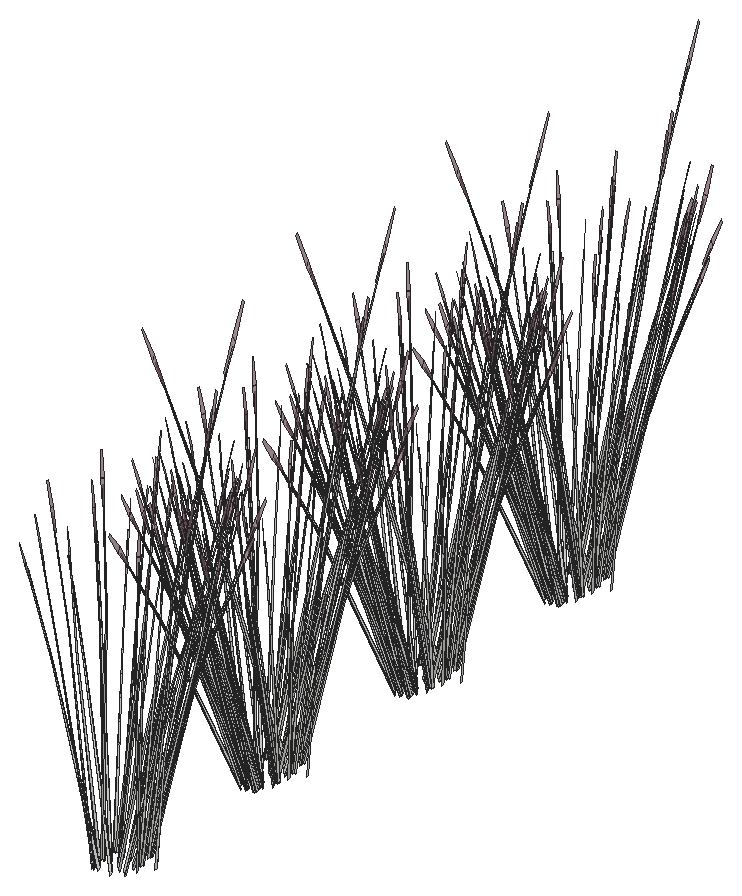
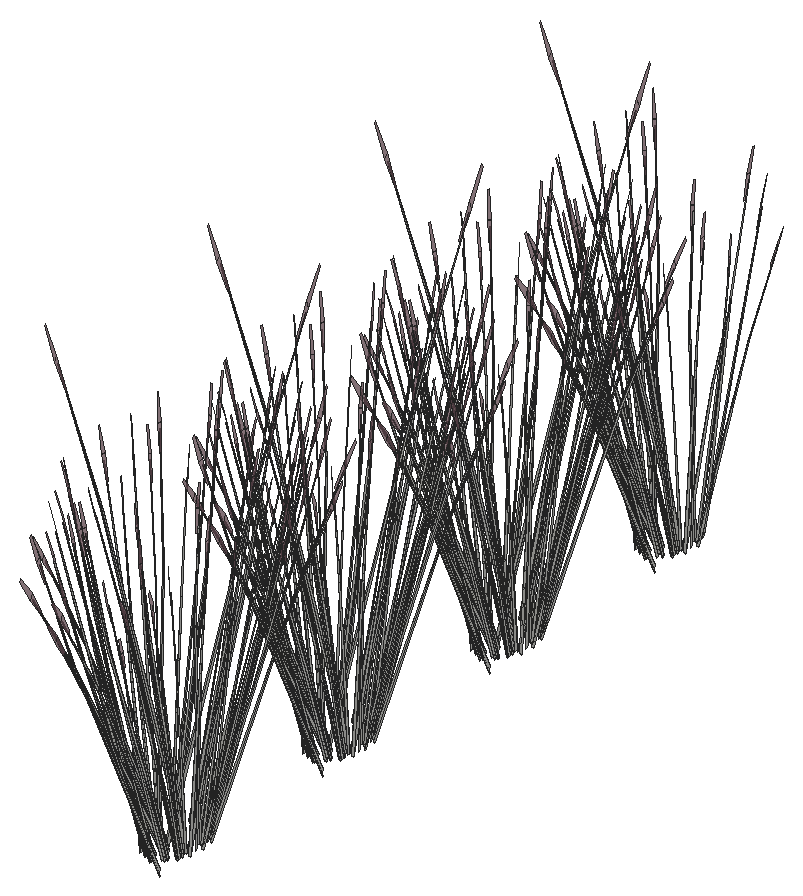
# SketchUp Ruby script. Lengths in inches.
U = 1.inch
M = Sketchup.active_model
def pt(a) = Geom::Point3d.new(a.map { |v| v * U })
def face(e, loops, mat)
  f = e.add_face(loops[0].map { |a| pt(a) })
  loops[1..].each { |l| e.add_face(l.map { |a| pt(a) }).erase! }
  f.material = f.back_material = mat if mat
  f
end
# faces: each face lists its corners as indices into pts; further lists are holes
def faces(e, pts, list, mat = nil) = list.each { |f| face(e, (f[0].is_a?(Array) ? f : [f]).map { |l| l.map { |i| pts[i] } }, mat) }
# xy, xz, yz: faces in a plane at the given z, y or x. An outline is a flat list of corners, or four numbers for a rectangle; further outlines are holes
def ring(l) = l.size == 4 ? [[l[0], l[1]], [l[2], l[1]], [l[2], l[3]], [l[0], l[3]]] : l.each_slice(2).to_a
def flat(e, list, mat, &to3) = list.each { |f| face(e, (f[0].is_a?(Array) ? f : [f]).map { |l| ring(l).map { |u, v| to3.(u, v) } }, mat) }
def xy(e, z, list, mat = nil) = flat(e, list, mat) { |x, y| [x, y, z] }
def xz(e, y, list, mat = nil) = flat(e, list, mat) { |x, z| [x, y, z] }
def yz(e, x, list, mat = nil) = flat(e, list, mat) { |y, z| [x, y, z] }
def lines(e, pts, list) = list.each { |a, b| e.add_line(pt(pts[a]), pt(pts[b])) }
# prism: a flat outline (further loops are holes) pulled along v
def prism(e, loops, v, mat = nil)
  f = face(e, loops, mat); d = Geom::Vector3d.new(v.map { |x| x * U })
  f.pushpull(f.normal.samedirection?(d) ? d.length : -d.length)
end
def box(e, o, s, mat = nil) = prism(e, [[o, [o[0] + s[0], o[1], o[2]], [o[0] + s[0], o[1] + s[1], o[2]], [o[0], o[1] + s[1], o[2]]]], [0, 0, s[2]], mat)
def at(x, y, z, deg = 0) = Geom::Transformation.translation(pt([x, y, z])) * Geom::Transformation.rotation(ORIGIN, Z_AXIS, deg.degrees)
def axes(o, x, y, z) = Geom::Transformation.new([*x, 0, *y, 0, *z, 0, *pt(o).to_a, 1])
def part(name) = M.definitions.add(name)
# library, detail: a bought-in or finely detailed component or shape, given as its bounding box
def library(name, o, s) = part(name).tap { |d| box(d.entities, o, s) }
def detail(e, o, s) = box(e.add_group.entities, o, s)
def put(e, d, t, mat = nil) = e.add_instance(d, t).tap { |i| i.material = mat if mat }
def group(e, t, mat = nil) = e.add_group.tap { |g| g.transformation = t; g.material = mat if mat }.entities
root = M.entities
M.materials.add("LightPink_Translucent").color = [144, 107, 117]
M.materials["LightPink_Translucent"].alpha = 0.75
c1 = part("blade")
p = [[2.15,0.21,22],[0,0.17,0],[0.09,0.45,0],[2.18,0.31,22],[2.29,0.31,22],[0.38,0.45,0],
  [2.48,0.24,33],[2.49,0.24,33],[2.48,0.22,33]]
faces(c1.entities,p,[[0,1,2,3],[4,5,2,3],[6,3,4,7],[8,0,3,6]])
c2 = part("seeds")
p = [[0.3,-0.1,1.38],[-0.01,-0.03,1.59],[-0.01,-0.03,0.03],[0.14,-0.07,-0.07],[0.29,-0.03,3],[0.15,0.01,3.11]]
faces(c2.entities,p,[[0,1,2,3],[1,0,4,5]],"LightPink_Translucent")
c3 = part("blade with seeds")
put(c3.entities,c1,at(0,0,0))
put(c3.entities,c2,axes([2.4,0.25,30.99],[1.5799,-0.05474,1.17369],[-0.12525,1.92788,0.29478],[-0.07173,-0.02425,1.56792]))
put(root,c3,axes([250.74,195.77,2.59],[-0.18586,0.40503,-0.37087],[-0.16277,-0.42787,-0.28727],[-0.09443,-0.06163,0.70962]))
put(root,c3,axes([250.84,195.35,2.85],[-0.0137,0.62183,-0.08826],[-0.25949,-0.017,-0.48986],[-0.09994,-0.0432,0.74434]))
put(root,c3,axes([252.78,197.73,2.85],[-0.12878,-0.55367,-0.08826],[0.22857,-0.27208,-0.48986],[0.09632,-0.07305,0.74434]))
put(root,c3,axes([252.77,197.26,2.59],[0.06934,-0.55619,-0.37087],[0.23774,0.19064,-0.28727],[0.09572,-0.051,0.70962]))
put(root,c3,axes([250.51,196.2,2.01],[0.10617,-0.01385,1.24382],[-0.07043,0.60021,0.10057],[-0.1513,-0.03712,0.53172]))
put(root,c3,axes([252.72,197.46,2.81],[0.22491,-0.27005,-0.51563],[0.12534,0.55588,0.06223],[0.10867,-0.06315,0.72942]))
put(root,c3,axes([252.91,197.51,2.48],[0.21272,0.17057,-0.25703],[-0.06204,0.49764,0.33183],[0.08564,-0.04563,0.63492]))
put(root,c3,axes([250.41,196.72,2.48],[-0.21272,-0.17057,-0.25703],[0.06204,-0.49764,0.33183],[-0.08564,0.04563,0.63492]))
put(root,c3,axes([252.33,196.9,2.01],[-0.10617,0.01385,1.24382],[0.07043,-0.60021,0.10057],[0.1513,0.03712,0.53172]))
put(root,c3,axes([251.0625,196.64,1.62],[0.07276,-0.08845,1.2851],[0.02509,0.61759,0.10057],[-0.15759,0.08195,0.4593]))
put(root,c3,axes([250.56,196.97,2.59],[-0.06934,0.55619,-0.37087],[-0.23774,-0.19064,-0.28727],[-0.09572,0.051,0.70962]))
put(root,c3,axes([250.55,196.5,2.85],[0.12878,0.55367,-0.08826],[-0.22857,0.27208,-0.48986],[-0.09632,0.07305,0.74434]))
put(root,c3,axes([253.09,198.9,2.04],[-0.04899,-0.514,-0.02534],[0.23154,-0.11817,-0.1149],[0.04835,0.03259,0.37899]))
put(root,c3,axes([252.49,198.88,2.85],[0.0137,-0.62183,-0.08826],[0.25949,0.017,-0.48986],[0.09994,0.0432,0.74434]))
put(root,c3,axes([250.55,197.26,2.01],[0.08881,-0.12933,1.24382],[0.07477,0.59764,0.10057],[-0.13942,0.13507,0.53172]))
put(root,c3,axes([252.5,198.58,2.81],[0.25586,0.01472,-0.51563],[-0.01718,0.61995,0.06223],[0.1084,0.06542,0.72942]))
put(root,c3,axes([252.66,198.84,2.48],[0.14563,0.38283,-0.25703],[-0.16629,0.3624,0.33183],[0.08449,0.05514,0.63492]))
put(root,c3,axes([250.49,198.15,2.48],[-0.2228,0.08739,-0.25703],[-0.05883,-0.49954,0.33183],[-0.06385,0.13418,0.63492]))
put(root,c3,axes([252.13,197.86,2.01],[-0.09507,-0.10535,1.24382],[0.19675,-0.44195,0.10057],[0.12263,0.19937,0.53172]))
put(root,c3,axes([252.15,196.47,2.44],[-0.22117,-0.3177,1.00363],[0.23354,-0.49464,0.43304],[0.07136,0.29809,0.97011]))
put(root,c3,axes([250.56,197.8125,2.85],[0.23676,0.33715,-0.08826],[-0.1364,0.48826,-0.48986],[-0.06689,0.16972,0.74434]))
put(root,c3,axes([251.98,199.56,2.85],[0.15252,-0.52338,-0.08826],[0.22088,0.30152,-0.48986],[0.07678,0.14787,0.74434]))
put(root,c3,axes([250.875,197.66,2.01],[0.06393,-0.18788,1.24382],[0.16142,0.50711,0.10057],[-0.11071,0.23094,0.53172]))
put(root,c3,axes([250.67,198.21,2.59],[0.06575,0.55831,-0.37087],[-0.24901,0.09767,-0.28727],[-0.07136,0.14996,0.70962]))
put(root,c3,axes([252.16,199.3,2.59],[0.25257,-0.14535,-0.37087],[0.04418,0.55045,-0.28727],[0.06784,0.15774,0.70962]))
put(root,c3,axes([250.83,198.125,2.01],[0.04766,-0.21017,1.24382],[0.19993,0.43493,0.10057],[-0.09019,0.27107,0.53172]))
put(root,c3,axes([250.88,199.31,2.48],[-0.17318,0.32193,-0.25703],[-0.16394,-0.36759,0.33183],[-0.02494,0.18677,0.63492]))
put(root,c3,axes([251.38,199.58,2.85],[0.25047,-0.28468,-0.08826],[0.12309,0.50526,-0.48986],[0.03305,0.21292,0.74434]))
put(root,c3,axes([251.06,199.16,2.83],[0.18323,0.41084,-0.41166],[-0.19356,0.3598,-0.31887],[-0.02788,0.20874,0.78768]))
put(root,c3,axes([251.6,199.56,2.59],[0.25161,0.15328,-0.37087],[-0.08624,0.52553,-0.28727],[0.02307,0.21159,0.70962]))
put(root,c3,axes([251.74,198.47,2.01],[-0.05851,-0.19632,1.24382],[0.27036,-0.16528,0.10057],[0.0611,0.3082,0.53172]))
put(root,c3,axes([251.48,199.88,2.48],[-0.07716,0.47021,-0.25703],[-0.22512,-0.13715,0.33183],[0.02064,0.18932,0.63492]))
put(root,c3,axes([251,198.97,3.07],[-0.00666,0.56559,-0.57235],[-0.28045,-0.03799,0.06907],[-0.0296,0.23961,0.80965]))
put(root,c3,axes([251.26,198.57,2.01],[-0.00626,-0.23468,1.24382],[0.27152,0.15569,0.10057],[-0.01679,0.33444,0.53172]))
put(root,c3,axes([251.51,199.46,2.81],[0.12216,0.49718,-0.51563],[-0.25147,0.27708,0.06223],[0.02857,0.24022,0.72942]))
put(root,c3,axes([251.1,209.88,2.01],[0.05851,0.19632,1.24382],[-0.27036,0.16528,0.10057],[-0.0611,-0.3082,0.53172]))
put(root,c3,axes([251.82,210.03,2.81],[-0.12216,-0.49718,-0.51563],[0.25147,-0.27708,0.06223],[-0.02857,-0.24022,0.72942]))
put(root,c3,axes([252.33,210.51,2.81],[0.00666,-0.56559,-0.51563],[0.28045,0.03799,0.06223],[0.0296,-0.23961,0.72942]))
put(root,c3,axes([250.9,199.77,1.63],[0.00562,-0.31565,1.12021],[0.25293,0.16673,0.1548],[-0.02192,0.33641,0.52896]))
put(root,c3,axes([251.84,209.6,2.48],[0.07716,-0.47021,-0.25703],[0.22512,0.13715,0.33183],[-0.02064,-0.18932,0.63492]))
put(root,c3,axes([252.01,210.23,2.01],[-0.04766,0.21017,1.24382],[-0.19993,-0.43493,0.10057],[0.09019,-0.27107,0.53172]))
put(root,c3,axes([251.73,209.93,2.59],[-0.25161,-0.15328,-0.37087],[0.08624,-0.52553,-0.28727],[-0.02307,-0.21159,0.70962]))
put(root,c3,axes([252.27,210.32,2.59],[-0.18323,-0.41084,-0.37087],[0.19356,-0.3598,-0.28727],[0.02788,-0.20874,0.70962]))
put(root,c3,axes([251.94,209.9,2.85],[-0.25047,0.28468,-0.08826],[-0.12309,-0.50526,-0.48986],[-0.03305,-0.21292,0.74434]))
put(root,c3,axes([252.46,210.54,2.85],[-0.2813,-0.0303,-0.08826],[0.00769,-0.57361,-0.48986],[0.01954,-0.22092,0.74434]))
put(root,c3,axes([252.44,210.17,2.48],[0.17318,-0.32193,-0.25703],[0.16394,0.36759,0.33183],[0.02494,-0.18677,0.63492]))
put(root,c3,axes([251.27,210.17,2.81],[-0.21825,-0.29555,-0.51563],[0.15511,-0.5179,0.06223],[-0.07907,-0.17646,0.72942]))
put(root,c3,axes([251.19,209.78,2.48],[-0.03953,-0.49251,-0.25703],[0.22598,-0.13005,0.33183],[-0.0607,-0.14114,0.63492]))
put(root,c3,axes([250.71,210.49,2.01],[0.09507,0.10535,1.24382],[-0.19675,0.44195,0.10057],[-0.12263,-0.19937,0.53172]))
put(root,c3,axes([251.17,210.18,2.59],[-0.25257,0.14535,-0.37087],[-0.04418,-0.55045,-0.28727],[-0.06784,-0.15774,0.70962]))
put(root,c3,axes([252.66,211.5,2.81],[0.1337,-0.48245,-0.51563],[0.23429,0.34287,0.06223],[0.07983,-0.1748,0.72942]))
put(root,c3,axes([252.65,211.27,2.59],[-0.06575,-0.55831,-0.37087],[0.24901,-0.09767,-0.28727],[0.07136,-0.14996,0.70962]))
put(root,c3,axes([252.77,211.67,2.85],[-0.23676,-0.33715,-0.08826],[0.1364,-0.48826,-0.48986],[0.06689,-0.16972,0.74434]))
put(root,c3,axes([251.79,213.51,1.61],[0.22119,0.24656,1.09782],[-0.21669,0.53118,0.43413],[-0.09706,-0.31482,0.92034]))
put(root,c3,axes([252.84,211.33,2.48],[0.2228,-0.08739,-0.25703],[0.05883,0.49954,0.33183],[0.06385,-0.13418,0.63492]))
put(root,c3,axes([250.67,210.64,2.48],[-0.14563,-0.38283,-0.25703],[0.16629,-0.3624,0.33183],[-0.08449,-0.05514,0.63492]))
put(root,c3,axes([250.82,210.9,2.81],[-0.25586,-0.01472,-0.51563],[0.01718,-0.61995,0.06223],[-0.1084,-0.06542,0.72942]))
put(root,c3,axes([250.74,211.02,2.59],[-0.18586,0.40503,-0.37087],[-0.16277,-0.42787,-0.28727],[-0.09443,-0.06163,0.70962]))
put(root,c3,axes([250.84,210.6,2.85],[-0.0137,0.62183,-0.08826],[-0.25949,-0.017,-0.48986],[-0.09994,-0.0432,0.74434]))
put(root,c3,axes([252.78,212.99,2.85],[-0.12878,-0.55367,-0.08826],[0.22857,-0.27208,-0.48986],[0.09632,-0.07305,0.74434]))
put(root,c3,axes([252.77,212.51,2.59],[0.06934,-0.55619,-0.37087],[0.23774,0.19064,-0.28727],[0.09572,-0.051,0.70962]))
put(root,c3,axes([250.51,211.46,2.01],[0.10617,-0.01385,1.24382],[-0.07043,0.60021,0.10057],[-0.1513,-0.03712,0.53172]))
put(root,c3,axes([252.72,212.71,2.81],[0.22491,-0.27005,-0.51563],[0.12534,0.55588,0.06223],[0.10867,-0.06315,0.72942]))
put(root,c3,axes([252.91,212.76,2.48],[0.21272,0.17057,-0.25703],[-0.06204,0.49764,0.33183],[0.08564,-0.04563,0.63492]))
put(root,c3,axes([250.41,211.97,2.48],[-0.21272,-0.17057,-0.25703],[0.06204,-0.49764,0.33183],[-0.08564,0.04563,0.63492]))
put(root,c3,axes([252.33,212.15,2.01],[-0.10617,0.01385,1.24382],[0.07043,-0.60021,0.10057],[0.1513,0.03712,0.53172]))
put(root,c3,axes([251.0625,211.89,1.62],[0.07276,-0.08845,1.2851],[0.02509,0.61759,0.10057],[-0.15759,0.08195,0.4593]))
put(root,c3,axes([250.56,212.23,2.59],[-0.06934,0.55619,-0.37087],[-0.23774,-0.19064,-0.28727],[-0.09572,0.051,0.70962]))
put(root,c3,axes([250.55,211.75,2.85],[0.12878,0.55367,-0.08826],[-0.22857,0.27208,-0.48986],[-0.09632,0.07305,0.74434]))
put(root,c3,axes([253.09,214.15,2.04],[-0.04899,-0.514,-0.02534],[0.23154,-0.11817,-0.1149],[0.04835,0.03259,0.37899]))
put(root,c3,axes([252.49,214.14,2.85],[0.0137,-0.62183,-0.08826],[0.25949,0.017,-0.48986],[0.09994,0.0432,0.74434]))
put(root,c3,axes([250.55,212.51,2.01],[0.08881,-0.12933,1.24382],[0.07477,0.59764,0.10057],[-0.13942,0.13507,0.53172]))
put(root,c3,axes([252.5,213.84,2.81],[0.25586,0.01472,-0.51563],[-0.01718,0.61995,0.06223],[0.1084,0.06542,0.72942]))
put(root,c3,axes([252.66,214.09,2.48],[0.14563,0.38283,-0.25703],[-0.16629,0.3624,0.33183],[0.08449,0.05514,0.63492]))
put(root,c3,axes([250.49,213.41,2.48],[-0.2228,0.08739,-0.25703],[-0.05883,-0.49954,0.33183],[-0.06385,0.13418,0.63492]))
put(root,c3,axes([252.13,213.11,2.01],[-0.09507,-0.10535,1.24382],[0.19675,-0.44195,0.10057],[0.12263,0.19937,0.53172]))
put(root,c3,axes([252.15,211.72,2.44],[-0.22117,-0.3177,1.00363],[0.23354,-0.49464,0.43304],[0.07136,0.29809,0.97011]))
put(root,c3,axes([250.56,213.07,2.85],[0.23676,0.33715,-0.08826],[-0.1364,0.48826,-0.48986],[-0.06689,0.16972,0.74434]))
put(root,c3,axes([251.98,214.8125,2.85],[0.15252,-0.52338,-0.08826],[0.22088,0.30152,-0.48986],[0.07678,0.14787,0.74434]))
put(root,c3,axes([250.875,212.91,2.01],[0.06393,-0.18788,1.24382],[0.16142,0.50711,0.10057],[-0.11071,0.23094,0.53172]))
put(root,c3,axes([250.67,213.46,2.59],[0.06575,0.55831,-0.37087],[-0.24901,0.09767,-0.28727],[-0.07136,0.14996,0.70962]))
put(root,c3,axes([252.16,214.55,2.59],[0.25257,-0.14535,-0.37087],[0.04418,0.55045,-0.28727],[0.06784,0.15774,0.70962]))
put(root,c3,axes([250.83,213.38,2.01],[0.04766,-0.21017,1.24382],[0.19993,0.43493,0.10057],[-0.09019,0.27107,0.53172]))
put(root,c3,axes([250.88,214.5625,2.48],[-0.17318,0.32193,-0.25703],[-0.16394,-0.36759,0.33183],[-0.02494,0.18677,0.63492]))
put(root,c3,axes([251.38,214.83,2.85],[0.25047,-0.28468,-0.08826],[0.12309,0.50526,-0.48986],[0.03305,0.21292,0.74434]))
put(root,c3,axes([251.06,214.41,2.83],[0.18323,0.41084,-0.41166],[-0.19356,0.3598,-0.31887],[-0.02788,0.20874,0.78768]))
put(root,c3,axes([251.6,214.81,2.59],[0.25161,0.15328,-0.37087],[-0.08624,0.52553,-0.28727],[0.02307,0.21159,0.70962]))
put(root,c3,axes([251.74,213.72,2.01],[-0.05851,-0.19632,1.24382],[0.27036,-0.16528,0.10057],[0.0611,0.3082,0.53172]))
put(root,c3,axes([251.48,215.13,2.48],[-0.07716,0.47021,-0.25703],[-0.22512,-0.13715,0.33183],[0.02064,0.18932,0.63492]))
put(root,c3,axes([251,214.22,3.07],[-0.00666,0.56559,-0.57235],[-0.28045,-0.03799,0.06907],[-0.0296,0.23961,0.80965]))
put(root,c3,axes([251.26,213.82,2.01],[-0.00626,-0.23468,1.24382],[0.27152,0.15569,0.10057],[-0.01679,0.33444,0.53172]))
put(root,c3,axes([251.51,214.71,2.81],[0.12216,0.49718,-0.51563],[-0.25147,0.27708,0.06223],[0.02857,0.24022,0.72942]))
put(root,c3,axes([251.1,225.39,2.01],[0.05851,0.19632,1.24382],[-0.27036,0.16528,0.10057],[-0.0611,-0.3082,0.53172]))
put(root,c3,axes([251.82,225.54,2.81],[-0.12216,-0.49718,-0.51563],[0.25147,-0.27708,0.06223],[-0.02857,-0.24022,0.72942]))
put(root,c3,axes([250.9,215.02,1.63],[0.00562,-0.31565,1.12021],[0.25293,0.16673,0.1548],[-0.02192,0.33641,0.52896]))
put(root,c3,axes([252.33,226.02,2.81],[0.00666,-0.56559,-0.51563],[0.28045,0.03799,0.06223],[0.0296,-0.23961,0.72942]))
put(root,c3,axes([251.84,225.11,2.48],[0.07716,-0.47021,-0.25703],[0.22512,0.13715,0.33183],[-0.02064,-0.18932,0.63492]))
put(root,c3,axes([252.01,225.74,2.01],[-0.04766,0.21017,1.24382],[-0.19993,-0.43493,0.10057],[0.09019,-0.27107,0.53172]))
put(root,c3,axes([251.73,225.4375,2.59],[-0.25161,-0.15328,-0.37087],[0.08624,-0.52553,-0.28727],[-0.02307,-0.21159,0.70962]))
put(root,c3,axes([252.27,225.83,2.59],[-0.18323,-0.41084,-0.37087],[0.19356,-0.3598,-0.28727],[0.02788,-0.20874,0.70962]))
put(root,c3,axes([251.94,225.41,2.85],[-0.25047,0.28468,-0.08826],[-0.12309,-0.50526,-0.48986],[-0.03305,-0.21292,0.74434]))
put(root,c3,axes([252.46,226.05,2.85],[-0.2813,-0.0303,-0.08826],[0.00769,-0.57361,-0.48986],[0.01954,-0.22092,0.74434]))
put(root,c3,axes([252.44,225.68,2.48],[0.17318,-0.32193,-0.25703],[0.16394,0.36759,0.33183],[0.02494,-0.18677,0.63492]))
put(root,c3,axes([251.27,225.68,2.81],[-0.21825,-0.29555,-0.51563],[0.15511,-0.5179,0.06223],[-0.07907,-0.17646,0.72942]))
put(root,c3,axes([251.19,225.29,2.48],[-0.03953,-0.49251,-0.25703],[0.22598,-0.13005,0.33183],[-0.0607,-0.14114,0.63492]))
put(root,c3,axes([250.71,226,2.01],[0.09507,0.10535,1.24382],[-0.19675,0.44195,0.10057],[-0.12263,-0.19937,0.53172]))
put(root,c3,axes([251.17,225.69,2.59],[-0.25257,0.14535,-0.37087],[-0.04418,-0.55045,-0.28727],[-0.06784,-0.15774,0.70962]))
put(root,c3,axes([252.66,227.01,2.81],[0.1337,-0.48245,-0.51563],[0.23429,0.34287,0.06223],[0.07983,-0.1748,0.72942]))
put(root,c3,axes([252.65,226.78,2.59],[-0.06575,-0.55831,-0.37087],[0.24901,-0.09767,-0.28727],[0.07136,-0.14996,0.70962]))
put(root,c3,axes([252.77,227.18,2.85],[-0.23676,-0.33715,-0.08826],[0.1364,-0.48826,-0.48986],[0.06689,-0.16972,0.74434]))
put(root,c3,axes([251.79,229.02,1.61],[0.22119,0.24656,1.09782],[-0.21669,0.53118,0.43413],[-0.09706,-0.31482,0.92034]))
put(root,c3,axes([252.84,226.84,2.48],[0.2228,-0.08739,-0.25703],[0.05883,0.49954,0.33183],[0.06385,-0.13418,0.63492]))
put(root,c3,axes([250.67,226.15,2.48],[-0.14563,-0.38283,-0.25703],[0.16629,-0.3624,0.33183],[-0.08449,-0.05514,0.63492]))
put(root,c3,axes([250.82,226.41,2.81],[-0.25586,-0.01472,-0.51563],[0.01718,-0.61995,0.06223],[-0.1084,-0.06542,0.72942]))
put(root,c3,axes([250.74,226.53,2.59],[-0.18586,0.40503,-0.37087],[-0.16277,-0.42787,-0.28727],[-0.09443,-0.06163,0.70962]))
put(root,c3,axes([250.84,226.11,2.85],[-0.0137,0.62183,-0.08826],[-0.25949,-0.017,-0.48986],[-0.09994,-0.0432,0.74434]))
put(root,c3,axes([252.78,228.5,2.85],[-0.12878,-0.55367,-0.08826],[0.22857,-0.27208,-0.48986],[0.09632,-0.07305,0.74434]))
put(root,c3,axes([252.77,228.02,2.59],[0.06934,-0.55619,-0.37087],[0.23774,0.19064,-0.28727],[0.09572,-0.051,0.70962]))
put(root,c3,axes([250.51,226.97,2.01],[0.10617,-0.01385,1.24382],[-0.07043,0.60021,0.10057],[-0.1513,-0.03712,0.53172]))
put(root,c3,axes([252.72,228.22,2.81],[0.22491,-0.27005,-0.51563],[0.12534,0.55588,0.06223],[0.10867,-0.06315,0.72942]))
put(root,c3,axes([252.91,228.27,2.48],[0.21272,0.17057,-0.25703],[-0.06204,0.49764,0.33183],[0.08564,-0.04563,0.63492]))
put(root,c3,axes([250.41,227.48,2.48],[-0.21272,-0.17057,-0.25703],[0.06204,-0.49764,0.33183],[-0.08564,0.04563,0.63492]))
put(root,c3,axes([252.33,227.66,2.01],[-0.10617,0.01385,1.24382],[0.07043,-0.60021,0.10057],[0.1513,0.03712,0.53172]))
put(root,c3,axes([251.0625,227.4,1.62],[0.07276,-0.08845,1.2851],[0.02509,0.61759,0.10057],[-0.15759,0.08195,0.4593]))
put(root,c3,axes([250.56,227.73,2.59],[-0.06934,0.55619,-0.37087],[-0.23774,-0.19064,-0.28727],[-0.09572,0.051,0.70962]))
put(root,c3,axes([250.55,227.26,2.85],[0.12878,0.55367,-0.08826],[-0.22857,0.27208,-0.48986],[-0.09632,0.07305,0.74434]))
put(root,c3,axes([253.09,229.66,2.04],[-0.04899,-0.514,-0.02534],[0.23154,-0.11817,-0.1149],[0.04835,0.03259,0.37899]))
put(root,c3,axes([252.49,229.65,2.85],[0.0137,-0.62183,-0.08826],[0.25949,0.017,-0.48986],[0.09994,0.0432,0.74434]))
put(root,c3,axes([250.55,228.02,2.01],[0.08881,-0.12933,1.24382],[0.07477,0.59764,0.10057],[-0.13942,0.13507,0.53172]))
put(root,c3,axes([252.5,229.35,2.81],[0.25586,0.01472,-0.51563],[-0.01718,0.61995,0.06223],[0.1084,0.06542,0.72942]))
put(root,c3,axes([252.66,229.6,2.48],[0.14563,0.38283,-0.25703],[-0.16629,0.3624,0.33183],[0.08449,0.05514,0.63492]))
put(root,c3,axes([250.49,228.92,2.48],[-0.2228,0.08739,-0.25703],[-0.05883,-0.49954,0.33183],[-0.06385,0.13418,0.63492]))
put(root,c3,axes([252.13,228.62,2.01],[-0.09507,-0.10535,1.24382],[0.19675,-0.44195,0.10057],[0.12263,0.19937,0.53172]))
put(root,c3,axes([252.15,227.23,2.44],[-0.22117,-0.3177,1.00363],[0.23354,-0.49464,0.43304],[0.07136,0.29809,0.97011]))
put(root,c3,axes([250.56,228.57,2.85],[0.23676,0.33715,-0.08826],[-0.1364,0.48826,-0.48986],[-0.06689,0.16972,0.74434]))
put(root,c3,axes([251.98,230.32,2.85],[0.15252,-0.52338,-0.08826],[0.22088,0.30152,-0.48986],[0.07678,0.14787,0.74434]))
put(root,c3,axes([250.875,228.42,2.01],[0.06393,-0.18788,1.24382],[0.16142,0.50711,0.10057],[-0.11071,0.23094,0.53172]))
put(root,c3,axes([250.67,228.97,2.59],[0.06575,0.55831,-0.37087],[-0.24901,0.09767,-0.28727],[-0.07136,0.14996,0.70962]))
put(root,c3,axes([252.16,230.0625,2.59],[0.25257,-0.14535,-0.37087],[0.04418,0.55045,-0.28727],[0.06784,0.15774,0.70962]))
put(root,c3,axes([250.83,228.89,2.01],[0.04766,-0.21017,1.24382],[0.19993,0.43493,0.10057],[-0.09019,0.27107,0.53172]))
put(root,c3,axes([250.88,230.07,2.48],[-0.17318,0.32193,-0.25703],[-0.16394,-0.36759,0.33183],[-0.02494,0.18677,0.63492]))
put(root,c3,axes([251.38,230.34,2.85],[0.25047,-0.28468,-0.08826],[0.12309,0.50526,-0.48986],[0.03305,0.21292,0.74434]))
put(root,c3,axes([251.06,229.92,2.83],[0.18323,0.41084,-0.41166],[-0.19356,0.3598,-0.31887],[-0.02788,0.20874,0.78768]))
put(root,c3,axes([251.6,230.32,2.59],[0.25161,0.15328,-0.37087],[-0.08624,0.52553,-0.28727],[0.02307,0.21159,0.70962]))
put(root,c3,axes([251.74,229.23,2.01],[-0.05851,-0.19632,1.24382],[0.27036,-0.16528,0.10057],[0.0611,0.3082,0.53172]))
put(root,c3,axes([251.48,230.64,2.48],[-0.07716,0.47021,-0.25703],[-0.22512,-0.13715,0.33183],[0.02064,0.18932,0.63492]))
put(root,c3,axes([251,229.73,3.07],[-0.00666,0.56559,-0.57235],[-0.28045,-0.03799,0.06907],[-0.0296,0.23961,0.80965]))
put(root,c3,axes([251.26,229.33,2.01],[-0.00626,-0.23468,1.24382],[0.27152,0.15569,0.10057],[-0.01679,0.33444,0.53172]))
put(root,c3,axes([251.1,240.47,2.01],[0.05851,0.19632,1.24382],[-0.27036,0.16528,0.10057],[-0.0611,-0.3082,0.53172]))
put(root,c3,axes([251.51,230.22,2.81],[0.12216,0.49718,-0.51563],[-0.25147,0.27708,0.06223],[0.02857,0.24022,0.72942]))
put(root,c3,axes([251.82,240.62,2.81],[-0.12216,-0.49718,-0.51563],[0.25147,-0.27708,0.06223],[-0.02857,-0.24022,0.72942]))
put(root,c3,axes([252.33,241.11,2.81],[0.00666,-0.56559,-0.51563],[0.28045,0.03799,0.06223],[0.0296,-0.23961,0.72942]))
put(root,c3,axes([251.84,240.2,2.48],[0.07716,-0.47021,-0.25703],[0.22512,0.13715,0.33183],[-0.02064,-0.18932,0.63492]))
put(root,c3,axes([252.01,240.82,2.01],[-0.04766,0.21017,1.24382],[-0.19993,-0.43493,0.10057],[0.09019,-0.27107,0.53172]))
put(root,c3,axes([250.9,230.53,1.63],[0.00562,-0.31565,1.12021],[0.25293,0.16673,0.1548],[-0.02192,0.33641,0.52896]))
put(root,c3,axes([251.73,240.52,2.59],[-0.25161,-0.15328,-0.37087],[0.08624,-0.52553,-0.28727],[-0.02307,-0.21159,0.70962]))
put(root,c3,axes([252.27,240.92,2.59],[-0.18323,-0.41084,-0.37087],[0.19356,-0.3598,-0.28727],[0.02788,-0.20874,0.70962]))
put(root,c3,axes([251.94,240.5,2.85],[-0.25047,0.28468,-0.08826],[-0.12309,-0.50526,-0.48986],[-0.03305,-0.21292,0.74434]))
put(root,c3,axes([252.46,241.13,2.85],[-0.2813,-0.0303,-0.08826],[0.00769,-0.57361,-0.48986],[0.01954,-0.22092,0.74434]))
put(root,c3,axes([252.44,240.77,2.48],[0.17318,-0.32193,-0.25703],[0.16394,0.36759,0.33183],[0.02494,-0.18677,0.63492]))
put(root,c3,axes([251.27,240.76,2.81],[-0.21825,-0.29555,-0.51563],[0.15511,-0.5179,0.06223],[-0.07907,-0.17646,0.72942]))
put(root,c3,axes([251.19,240.37,2.48],[-0.03953,-0.49251,-0.25703],[0.22598,-0.13005,0.33183],[-0.0607,-0.14114,0.63492]))
put(root,c3,axes([250.71,241.09,2.01],[0.09507,0.10535,1.24382],[-0.19675,0.44195,0.10057],[-0.12263,-0.19937,0.53172]))
put(root,c3,axes([251.17,240.78,2.59],[-0.25257,0.14535,-0.37087],[-0.04418,-0.55045,-0.28727],[-0.06784,-0.15774,0.70962]))
put(root,c3,axes([252.66,242.09,2.81],[0.1337,-0.48245,-0.51563],[0.23429,0.34287,0.06223],[0.07983,-0.1748,0.72942]))
put(root,c3,axes([252.65,241.86,2.59],[-0.06575,-0.55831,-0.37087],[0.24901,-0.09767,-0.28727],[0.07136,-0.14996,0.70962]))
put(root,c3,axes([252.77,242.26,2.85],[-0.23676,-0.33715,-0.08826],[0.1364,-0.48826,-0.48986],[0.06689,-0.16972,0.74434]))
put(root,c3,axes([251.79,244.1,1.61],[0.22119,0.24656,1.09782],[-0.21669,0.53118,0.43413],[-0.09706,-0.31482,0.92034]))
put(root,c3,axes([252.84,241.92,2.48],[0.2228,-0.08739,-0.25703],[0.05883,0.49954,0.33183],[0.06385,-0.13418,0.63492]))
put(root,c3,axes([250.67,241.24,2.48],[-0.14563,-0.38283,-0.25703],[0.16629,-0.3624,0.33183],[-0.08449,-0.05514,0.63492]))
put(root,c3,axes([250.82,241.49,2.81],[-0.25586,-0.01472,-0.51563],[0.01718,-0.61995,0.06223],[-0.1084,-0.06542,0.72942]))
put(root,c3,axes([250.74,241.62,2.59],[-0.18586,0.40503,-0.37087],[-0.16277,-0.42787,-0.28727],[-0.09443,-0.06163,0.70962]))
put(root,c3,axes([250.84,241.19,2.85],[-0.0137,0.62183,-0.08826],[-0.25949,-0.017,-0.48986],[-0.09994,-0.0432,0.74434]))
put(root,c3,axes([252.78,243.58,2.85],[-0.12878,-0.55367,-0.08826],[0.22857,-0.27208,-0.48986],[0.09632,-0.07305,0.74434]))
put(root,c3,axes([252.77,243.1,2.59],[0.06934,-0.55619,-0.37087],[0.23774,0.19064,-0.28727],[0.09572,-0.051,0.70962]))
put(root,c3,axes([250.51,242.05,2.01],[0.10617,-0.01385,1.24382],[-0.07043,0.60021,0.10057],[-0.1513,-0.03712,0.53172]))
put(root,c3,axes([252.72,243.31,2.81],[0.22491,-0.27005,-0.51563],[0.12534,0.55588,0.06223],[0.10867,-0.06315,0.72942]))
put(root,c3,axes([252.91,243.36,2.48],[0.21272,0.17057,-0.25703],[-0.06204,0.49764,0.33183],[0.08564,-0.04563,0.63492]))
put(root,c3,axes([250.41,242.57,2.48],[-0.21272,-0.17057,-0.25703],[0.06204,-0.49764,0.33183],[-0.08564,0.04563,0.63492]))
put(root,c3,axes([252.33,242.74,2.01],[-0.10617,0.01385,1.24382],[0.07043,-0.60021,0.10057],[0.1513,0.03712,0.53172]))
put(root,c3,axes([251.0625,242.48,1.62],[0.07276,-0.08845,1.2851],[0.02509,0.61759,0.10057],[-0.15759,0.08195,0.4593]))
put(root,c3,axes([250.56,242.82,2.59],[-0.06934,0.55619,-0.37087],[-0.23774,-0.19064,-0.28727],[-0.09572,0.051,0.70962]))
put(root,c3,axes([250.55,242.34,2.85],[0.12878,0.55367,-0.08826],[-0.22857,0.27208,-0.48986],[-0.09632,0.07305,0.74434]))
put(root,c3,axes([253.09,244.75,2.04],[-0.04899,-0.514,-0.02534],[0.23154,-0.11817,-0.1149],[0.04835,0.03259,0.37899]))
put(root,c3,axes([252.49,244.73,2.85],[0.0137,-0.62183,-0.08826],[0.25949,0.017,-0.48986],[0.09994,0.0432,0.74434]))
put(root,c3,axes([250.55,243.11,2.01],[0.08881,-0.12933,1.24382],[0.07477,0.59764,0.10057],[-0.13942,0.13507,0.53172]))
put(root,c3,axes([252.5,244.43,2.81],[0.25586,0.01472,-0.51563],[-0.01718,0.61995,0.06223],[0.1084,0.06542,0.72942]))
put(root,c3,axes([252.66,244.6875,2.48],[0.14563,0.38283,-0.25703],[-0.16629,0.3624,0.33183],[0.08449,0.05514,0.63492]))
put(root,c3,axes([250.49,244,2.48],[-0.2228,0.08739,-0.25703],[-0.05883,-0.49954,0.33183],[-0.06385,0.13418,0.63492]))
put(root,c3,axes([252.13,243.71,2.01],[-0.09507,-0.10535,1.24382],[0.19675,-0.44195,0.10057],[0.12263,0.19937,0.53172]))
put(root,c3,axes([252.15,242.32,2.44],[-0.22117,-0.3177,1.00363],[0.23354,-0.49464,0.43304],[0.07136,0.29809,0.97011]))
put(root,c3,axes([250.56,243.66,2.85],[0.23676,0.33715,-0.08826],[-0.1364,0.48826,-0.48986],[-0.06689,0.16972,0.74434]))
put(root,c3,axes([251.98,245.41,2.85],[0.15252,-0.52338,-0.08826],[0.22088,0.30152,-0.48986],[0.07678,0.14787,0.74434]))
put(root,c3,axes([250.875,243.51,2.01],[0.06393,-0.18788,1.24382],[0.16142,0.50711,0.10057],[-0.11071,0.23094,0.53172]))
put(root,c3,axes([250.67,244.06,2.59],[0.06575,0.55831,-0.37087],[-0.24901,0.09767,-0.28727],[-0.07136,0.14996,0.70962]))
put(root,c3,axes([252.16,245.15,2.59],[0.25257,-0.14535,-0.37087],[0.04418,0.55045,-0.28727],[0.06784,0.15774,0.70962]))
put(root,c3,axes([250.83,243.97,2.01],[0.04766,-0.21017,1.24382],[0.19993,0.43493,0.10057],[-0.09019,0.27107,0.53172]))
put(root,c3,axes([250.88,245.16,2.48],[-0.17318,0.32193,-0.25703],[-0.16394,-0.36759,0.33183],[-0.02494,0.18677,0.63492]))
put(root,c3,axes([251.38,245.43,2.85],[0.25047,-0.28468,-0.08826],[0.12309,0.50526,-0.48986],[0.03305,0.21292,0.74434]))
put(root,c3,axes([251.06,245,2.83],[0.18323,0.41084,-0.41166],[-0.19356,0.3598,-0.31887],[-0.02788,0.20874,0.78768]))
put(root,c3,axes([251.6,245.4,2.59],[0.25161,0.15328,-0.37087],[-0.08624,0.52553,-0.28727],[0.02307,0.21159,0.70962]))
put(root,c3,axes([251.74,244.32,2.01],[-0.05851,-0.19632,1.24382],[0.27036,-0.16528,0.10057],[0.0611,0.3082,0.53172]))
put(root,c3,axes([251.48,245.72,2.48],[-0.07716,0.47021,-0.25703],[-0.22512,-0.13715,0.33183],[0.02064,0.18932,0.63492]))
put(root,c3,axes([251,244.82,3.07],[-0.00666,0.56559,-0.57235],[-0.28045,-0.03799,0.06907],[-0.0296,0.23961,0.80965]))
put(root,c3,axes([251.26,244.42,2.01],[-0.00626,-0.23468,1.24382],[0.27152,0.15569,0.10057],[-0.01679,0.33444,0.53172]))
put(root,c3,axes([251.51,245.3,2.81],[0.12216,0.49718,-0.51563],[-0.25147,0.27708,0.06223],[0.02857,0.24022,0.72942]))
put(root,c3,axes([250.9,245.61,1.63],[0.00562,-0.31565,1.12021],[0.25293,0.16673,0.1548],[-0.02192,0.33641,0.52896]))
